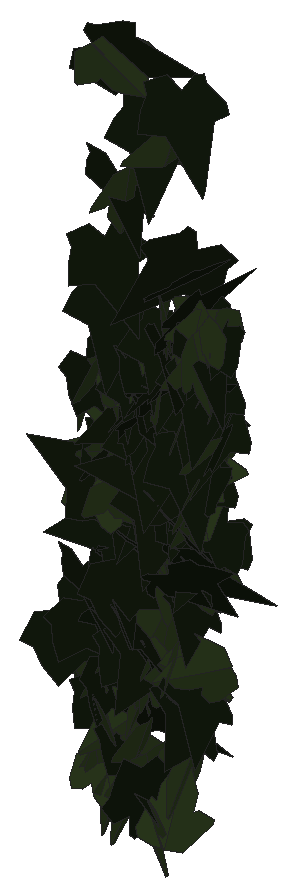
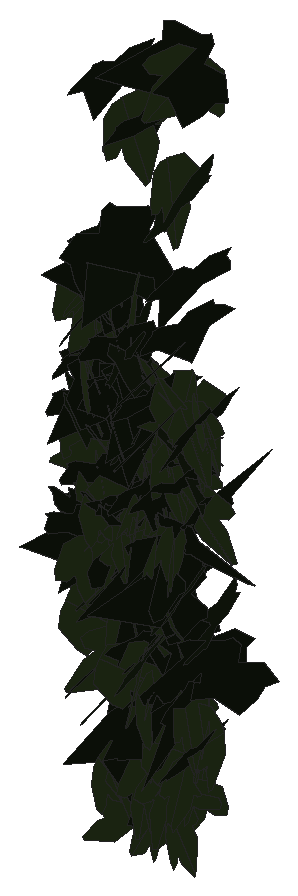
# SketchUp Ruby script. Lengths in inches.
U = 1.inch
M = Sketchup.active_model
def pt(a) = Geom::Point3d.new(a.map { |v| v * U })
def face(e, loops, mat)
  f = e.add_face(loops[0].map { |a| pt(a) })
  loops[1..].each { |l| e.add_face(l.map { |a| pt(a) }).erase! }
  f.material = f.back_material = mat if mat
  f
end
# faces: each face lists its corners as indices into pts; further lists are holes
def faces(e, pts, list, mat = nil) = list.each { |f| face(e, (f[0].is_a?(Array) ? f : [f]).map { |l| l.map { |i| pts[i] } }, mat) }
# xy, xz, yz: faces in a plane at the given z, y or x. An outline is a flat list of corners, or four numbers for a rectangle; further outlines are holes
def ring(l) = l.size == 4 ? [[l[0], l[1]], [l[2], l[1]], [l[2], l[3]], [l[0], l[3]]] : l.each_slice(2).to_a
def flat(e, list, mat, &to3) = list.each { |f| face(e, (f[0].is_a?(Array) ? f : [f]).map { |l| ring(l).map { |u, v| to3.(u, v) } }, mat) }
def xy(e, z, list, mat = nil) = flat(e, list, mat) { |x, y| [x, y, z] }
def xz(e, y, list, mat = nil) = flat(e, list, mat) { |x, z| [x, y, z] }
def yz(e, x, list, mat = nil) = flat(e, list, mat) { |y, z| [x, y, z] }
def lines(e, pts, list) = list.each { |a, b| e.add_line(pt(pts[a]), pt(pts[b])) }
# prism: a flat outline (further loops are holes) pulled along v
def prism(e, loops, v, mat = nil)
  f = face(e, loops, mat); d = Geom::Vector3d.new(v.map { |x| x * U })
  f.pushpull(f.normal.samedirection?(d) ? d.length : -d.length)
end
def box(e, o, s, mat = nil) = prism(e, [[o, [o[0] + s[0], o[1], o[2]], [o[0] + s[0], o[1] + s[1], o[2]], [o[0], o[1] + s[1], o[2]]]], [0, 0, s[2]], mat)
def at(x, y, z, deg = 0) = Geom::Transformation.translation(pt([x, y, z])) * Geom::Transformation.rotation(ORIGIN, Z_AXIS, deg.degrees)
def axes(o, x, y, z) = Geom::Transformation.new([*x, 0, *y, 0, *z, 0, *pt(o).to_a, 1])
def part(name) = M.definitions.add(name)
# library, detail: a bought-in or finely detailed component or shape, given as its bounding box
def library(name, o, s) = part(name).tap { |d| box(d.entities, o, s) }
def detail(e, o, s) = box(e.add_group.entities, o, s)
def put(e, d, t, mat = nil) = e.add_instance(d, t).tap { |i| i.material = mat if mat }
def group(e, t, mat = nil) = e.add_group.tap { |g| g.transformation = t; g.material = mat if mat }.entities
root = M.entities
M.materials.add("efeu1").color = [18, 25, 13]
M.materials.add("efeu2").color = [43, 57, 29]
c1 = part("ivyleaf_9")
p = [[1.54,2.16,1.25],[1.36,2.04,1.19],[-0.21,0.99,0.68],[-0.71,1.11,0.82],[-0.85,0.86,0.67],[-0.8,0.17,0.21],
  [-0.9,-0.01,0.1],[-0.67,-0.16,-0.02],[-0.08,-0.08,-0.05],[-0.03,-0.6,-0.4],[0.65,-0.88,-0.66],[0.83,-0.6,-0.49],
  [1.29,-0.42,-0.43],[1.8125,-0.07,-0.26],[1.21,0.44,0.15]]
faces(c1.entities,p,[[0,1,2,3,4,5,6,7,8,9,10,11,12,13,14]],"efeu1")
c2 = part("ivyleaf_10")
p = [[0,0.5,-0.03],[-0.0625,2.02,-0.43],[-0.19,2.01,-0.46],[-0.54,1.05,-0.29],[-0.52,0.625,-0.18],[-0.83,0.76,-0.28],
  [-1.16,0.64,-0.33],[-1.15,0.33,-0.24],[-0.77,-0.39,0.02],[-0.3,-0.51,0.16],[0.04,-0.48,0.23],[-0.02,2.01,-0.4375],
  [-0.06,2.01,-0.43],[0.04,-0.49,0.23],[0.67,-0.49,0.14],[1.38,0.36,-0.2],[1.375,0.51,-0.24],[0.81,0.65,-0.19],
  [0.62,0.59,-0.15],[0.6,1.09,-0.28],[0.5,1.23,-0.31]]
faces(c2.entities,p,[[0,1,2,3,4,5,6,7,8,9,10],[11,12,0,13,14,15,16,17,18,19,20]],"efeu2")
put(root,c1,axes([527.8,135.33,192.03],[-0.03574,-0.7717,-0.11443],[0.021,-0.11546,0.77209],[-0.77985,0.03225,0.02603]))
put(root,c2,axes([528.8125,134.72,192.54],[-0.44969,-0.49073,-0.36968],[0.25288,0.26967,-0.6656],[0.55993,-0.5159,0.00372]))
put(root,c1,axes([529.75,135.24,194.07],[-0.50214,-0.56983,-0.24591],[0.18261,0.16666,-0.75908],[0.59315,-0.53371,0.02551]))
put(root,c1,axes([529.15,135.53,188.14],[-0.1899,-0.62733,0.39079],[-0.02208,-0.39849,-0.65041],[0.73876,-0.17316,0.08101]))
put(root,c1,axes([530.28,135.32,192.99],[-0.40472,-0.05704,0.74689],[-0.72954,-0.16255,-0.40773],[0.16991,-0.8338,0.02839]))
put(root,c1,axes([530.52,135.21,193.8125],[0.00337,-0.78001,-0.14313],[0.01316,0.14317,-0.7799],[0.79293,0.00094,0.01355]))
put(root,c2,axes([529.96,135.16,201.61],[-0.17501,-0.81085,0.17773],[-0.03106,-0.17511,-0.8295],[0.82952,-0.17762,0.00644]))
put(root,c1,axes([530.56,134.53,190.9],[0.64926,0.46368,0.09757],[0.0766,0.06063,-0.79782],[-0.4676,0.65375,0.00479]))
put(root,c1,axes([529.5,135.23,191.96],[0.37439,-0.43591,0.54064],[0.42975,-0.33705,-0.56937],[0.54555,0.56467,0.0775]))
put(root,c2,axes([531.26,135.26,188.42],[-0.21255,-0.15598,0.72531],[-0.58518,-0.42853,-0.26365],[0.45604,-0.62259,-0.00025]))
put(root,c1,axes([529.3125,135.04,194.65],[-0.69836,0.30086,0.13229],[-0.12525,0.04361,-0.76035],[-0.30386,-0.70944,0.00936]))
put(root,c1,axes([529.4,135.41,201.91],[-0.07236,-0.80977,0.03417],[0.00042,-0.03434,-0.81298],[0.81049,-0.07228,0.00347]))
put(root,c2,axes([528.15,134.8125,186.65],[-0.56665,0.37683,0.32052],[-0.27282,0.16852,-0.68044],[-0.41268,-0.62883,0.00972]))
put(root,c2,axes([528.79,135.09,200.41],[-0.01641,-0.81,-0.0689],[0.01851,0.06853,-0.80999],[0.81271,-0.01792,0.01705]))
put(root,c2,axes([529.46,135.15,195.1875],[0.62857,-0.48335,-0.03124],[-0.01441,0.0325,-0.79274],[0.48415,0.62851,0.01697]))
put(root,c1,axes([528.2,135.48,189.92],[0.22228,-0.68125,0.31969],[0.12627,-0.29486,-0.71612],[0.74186,0.25431,0.0261]))
put(root,c2,axes([528.87,135.4,184.65],[0.09663,-0.71428,0.33007],[0.05891,-0.32505,-0.72066],[0.78465,0.11237,0.01346]))
put(root,c1,axes([528.18,135.52,200.06],[0.20878,-0.72157,0.37063],[0.22611,-0.31578,-0.74215],[0.77905,0.28503,0.11607]))
put(root,c1,axes([527.26,135.44,189.51],[0.33011,-0.63873,0.28091],[0.15388,-0.23647,-0.71852],[0.6806,0.36327,0.02621]))
put(root,c1,axes([529.67,135.69,195.72],[0.08238,-0.52453,0.64775],[0.19724,-0.62015,-0.52726],[0.80982,0.2044,0.06253]))
put(root,c1,axes([528.21,135.5,196.98],[-0.16926,-0.77638,-0.03937],[-0.00605,0.04161,-0.79448],[0.77735,-0.16873,-0.01476]))
put(root,c2,axes([528.55,135.12,192.94],[-0.7037,-0.23781,0.16983],[-0.15629,-0.06789,-0.74267],[0.24691,-0.72071,0.01392]))
put(root,c1,axes([528.42,135.22,185.6],[0.47955,-0.61319,-0.08546],[-0.04016,0.07706,-0.77828],[0.61781,0.48098,0.01574]))
put(root,c2,axes([529.01,135.33,185.88],[0.1496,-0.73188,0.13676],[0.02028,-0.13544,-0.74698],[0.74427,0.1508,-0.00714]))
put(root,c2,axes([530.97,134.96,196.69],[-0.02522,0.77112,0.12282],[-0.07199,0.12006,-0.7686],[-0.77751,-0.03613,0.06718]))
put(root,c2,axes([530.94,135.2,197.25],[-0.6481,0.13698,0.41878],[-0.44061,-0.2064,-0.61436],[0.00291,-0.74351,0.2477]))
put(root,c1,axes([528.87,135.18,189.05],[0.53224,-0.54154,-0.08727],[-0.03394,0.08886,-0.75837],[0.54748,0.53198,0.03783]))
put(root,c1,axes([528.63,134.71,193.51],[-0.18466,0.65837,0.36688],[-0.17846,0.3288,-0.67985],[-0.73226,-0.24616,0.07316]))
put(root,c1,axes([530.18,135.77,186.69],[-0.14093,-0.58061,0.4936],[0.04433,-0.50736,-0.58415],[0.76078,-0.07799,0.12547]))
put(root,c1,axes([530.22,135.33,202.95],[0.02757,-0.77223,-0.27105],[-0.00509,0.27104,-0.77271],[0.8184,0.0277,0.00433]))
put(root,c2,axes([527.68,135.34,194.95],[0.30123,-0.76115,0.04639],[0.00648,-0.04732,-0.81852],[0.76254,0.30109,-0.01137]))
put(root,c1,axes([529.29,134.66,184.28],[-0.0796,-0.05712,0.82665],[0.53853,0.62759,0.09522],[-0.62976,0.54389,-0.02306]))
put(root,c1,axes([529.5625,135.63,192.18],[-0.27612,-0.72698,0.016],[-0.00639,-0.01468,-0.77765],[0.72713,-0.2762,-0.00076]))
put(root,c1,axes([529.32,135.51,194.09],[0.38919,-0.65365,0.20644],[0.10684,-0.17665,-0.76074],[0.6771,0.40358,0.00138]))
put(root,c1,axes([529.83,135.41,195.76],[-0.6008,0.40455,-0.30162],[0.15522,-0.29809,-0.70898],[-0.48015,-0.60256,0.14822]))
put(root,c1,axes([528.67,135.3,191.36],[-0.65059,0.20394,0.39045],[-0.38126,0.08812,-0.68131],[-0.22064,-0.75363,0.02599]))
put(root,c2,axes([530.72,135.125,192.99],[0.21409,-0.69798,-0.30106],[-0.09706,0.28512,-0.73003],[0.75392,0.23491,-0.00849]))
put(root,c1,axes([528.82,135.125,189.24],[0.29871,0.59046,-0.43472],[-0.1676,-0.402,-0.66118],[-0.71382,0.34147,-0.02668]))
put(root,c2,axes([528.78,135.74,187.31],[-0.23096,-0.13339,0.70643],[0.49844,-0.56441,0.05638],[0.51807,0.48356,0.26069]))
put(root,c1,axes([527.98,135.33,198.36],[0.12095,-0.72043,-0.33191],[-0.00905,0.33448,-0.72929],[0.79316,0.11367,0.04229]))
put(root,c2,axes([529.62,135.37,187.98],[-0.62672,-0.06817,0.37557],[-0.33347,-0.25357,-0.60248],[0.18575,-0.68522,0.18558]))
put(root,c2,axes([528.01,135.2,184.92],[0.62327,0.30802,0.18403],[0.13473,0.14096,-0.69223],[-0.33255,0.6344,0.06446]))
put(root,c1,axes([530.4,135.75,187.49],[0.01709,-0.72583,0.23978],[0.06211,-0.23773,-0.72405],[0.76188,0.03566,0.05365]))
put(root,c2,axes([528.49,135.77,186.08],[-0.19638,-0.27838,0.66925],[-0.1969,-0.64681,-0.32682],[0.69758,-0.26094,0.09615]))
put(root,c1,axes([530.08,135.8,189.84],[0.01547,-0.69659,0.34377],[0.11071,-0.33835,-0.69059],[0.76887,0.06274,0.09253]))
put(root,c2,axes([528.16,135.1,203.41],[-0.61065,-0.2846,-0.48513],[0.4563,0.16799,-0.67291],[0.32884,-0.76159,0.03286]))
put(root,c2,axes([530.76,135.375,196.18],[-0.16071,-0.7675,0.0093],[0.05542,-0.02108,-0.78196],[0.76555,-0.15959,0.05856]))
put(root,c2,axes([529.125,135.32,183.92],[-0.54492,0.40266,-0.30524],[0.24575,-0.18104,-0.67755],[-0.44149,-0.59777,-0.00041]))
put(root,c1,axes([530.65,135.76,195.65],[-0.13892,-0.7766,0.1023],[0.00037,-0.10396,-0.78871],[0.78331,-0.13768,0.01851]))
put(root,c1,axes([530.24,135.72,198.67],[-0.07385,0.24379,-0.83335],[-0.04121,-0.8364,-0.24103],[-0.8673,0.01899,0.08241]))
put(root,c2,axes([527.29,135.47,186.63],[-0.46161,0.35338,-0.58612],[0.46446,-0.35751,-0.58135],[-0.50268,-0.65484,0.00108]))
put(root,c2,axes([529.75,135.23,197.25],[-0.49673,0.63448,0.0429],[-0.13759,-0.05409,-0.79328],[-0.62087,-0.49564,0.14148]))
put(root,c1,axes([528.8,134.82,190.55],[0.29483,-0.24248,-0.87086],[-0.01335,0.91474,-0.25922],[0.90389,0.0926,0.28023]))
put(root,c1,axes([528.95,135.73,194.99],[-0.17651,-0.75548,0.0174],[-0.00445,-0.01683,-0.77582],[0.75566,-0.17656,-0.00051]))
put(root,c2,axes([529.47,135.49,188.99],[-0.50086,-0.48174,0.2918],[-0.19998,-0.21293,-0.6948],[0.52652,-0.53913,0.01368]))
put(root,c2,axes([530.94,135.54,197.15],[-0.34051,-0.70121,0.17409],[0.05839,-0.21853,-0.76602],[0.72014,-0.31385,0.14443]))
put(root,c2,axes([530.03,135.16,188.7],[0.40823,-0.5559,-0.49614],[-0.30105,0.39444,-0.68965],[0.68158,0.50718,-0.00745]))
put(root,c1,axes([530.57,135.65,196.76],[0.2515,-0.75774,0.05383],[0.00247,-0.05589,-0.79824],[0.75965,0.25105,-0.01522]))
put(root,c2,axes([528.37,135.21,194.74],[0.68537,-0.10734,0.38785],[-0.37697,0.09688,0.69296],[-0.14086,-0.78152,0.03263]))
put(root,c1,axes([528.62,135.14,188.43],[0.6498,0.10918,-0.4395],[-0.43013,-0.09161,-0.65872],[-0.14163,0.7791,-0.01587]))
put(root,c2,axes([528.6,134.97,192.38],[0.35563,0.39365,0.6463],[0.35924,0.54069,-0.52701],[-0.66604,0.50182,0.06084]))
put(root,c2,axes([528.74,135.5,191.49],[-0.55508,0.30851,-0.44186],[0.32425,-0.31547,-0.62759],[-0.43044,-0.63548,0.09704]))
put(root,c1,axes([527.59,135.11,188.875],[-0.00469,-0.3709,-0.69976],[0.03675,0.69891,-0.3707],[0.79112,-0.03466,0.01307]))
put(root,c2,axes([528.04,135.29,194.47],[0.65068,-0.35549,-0.26657],[-0.14985,0.26945,-0.72509],[0.4183,0.6495,0.15491]))
put(root,c1,axes([529.46,134.81,194.62],[0.27935,0.64425,0.33928],[0.12309,0.31637,-0.70211],[-0.71764,0.30504,0.01164]))
put(root,c2,axes([529.08,135.3125,193.42],[0.53184,-0.50481,-0.2839],[-0.13896,0.26295,-0.72789],[0.56224,0.54251,0.08864]))
put(root,c1,axes([528.01,135.02,203.5625],[0.16967,0.23859,-0.77992],[0.44244,0.64229,0.29274],[0.68516,-0.47384,0.0041]))
put(root,c2,axes([527.83,135.46,192.5],[0.67893,-0.09891,-0.43903],[-0.4333,0.07104,-0.68606],[0.1216,0.80538,0.0066]))
put(root,c2,axes([529.36,135.3,190.87],[-0.62429,0.42429,0.02489],[-0.0211,0.01322,-0.75482],[-0.4245,-0.62464,0.00093]))
put(root,c2,axes([530.85,135.63,195.4],[0.5442,-0.57311,0.1023],[0.05742,-0.08651,-0.79012],[0.57933,0.54693,-0.01779]))
put(root,c2,axes([530.04,135.06,190.37],[-0.12901,0.63164,0.40942],[-0.13435,0.38939,-0.64309],[-0.74064,-0.18066,0.04534]))
put(root,c1,axes([526.98,135.09,188.48],[0.26067,-0.27434,-0.85378],[0.2872,0.86783,-0.19116],[0.84954,-0.20921,0.3266]))
put(root,c1,axes([530.87,135.06,192.67],[-0.72338,0.34776,-0.12421],[-0.11613,0.04509,0.80258],[0.35054,0.73258,0.00956]))
put(root,c1,axes([530.35,134.85,197.2],[-0.09302,0.65707,-0.46318],[-0.09984,0.45322,0.66299],[0.79769,0.13335,0.02897]))
put(root,c1,axes([530.2,135.32,190.64],[0.62236,-0.07483,0.49451],[0.49263,-0.04458,-0.62674],[0.08635,0.79365,0.01142]))
put(root,c2,axes([528.78,135.97,187.24],[0.1445,-0.54934,0.56919],[0.26502,-0.51155,-0.56099],[0.74533,0.2884,0.08912]))
put(root,c1,axes([531.12,135.71,197],[-0.75984,0.03985,-0.22383],[0.22384,-0.00565,-0.76086],[-0.03982,-0.7921,-0.00583]))
put(root,c2,axes([528.18,135.35,194],[0.75951,0.16265,-0.27372],[0.26857,0.05298,0.77672],[0.17101,-0.80558,-0.00418]))
put(root,c2,axes([529.85,135.74,194.0625],[0.43704,-0.62924,0.18954],[0.1091,-0.155,-0.76612],[0.64805,0.45045,0.00115]))
put(root,c1,axes([529.67,135.875,196.27],[-0.37369,-0.68913,-0.10923],[0.06432,0.08936,-0.78381],[0.69476,-0.37893,0.01381]))
put(root,c2,axes([529.24,135.46,193.21],[0.37908,-0.62975,-0.27747],[-0.15115,0.23285,-0.73499],[0.67136,0.408,-0.00881]))
put(root,c1,axes([530.65,135.93,194.58],[-0.40838,-0.67211,-0.04345],[0.01731,0.04032,-0.78643],[0.67329,-0.4087,-0.00614]))
put(root,c2,axes([527.92,135.59,187.25],[0.09212,-0.74944,-0.06245],[-0.00056,0.06285,-0.75505],[0.75204,0.09185,0.00709]))
put(root,c1,axes([528.57,135.43,190.47],[0.73295,-0.16802,0.24714],[0.24013,-0.05855,-0.75196],[0.1779,0.77128,-0.00324]))
put(root,c2,axes([528.31,135.6875,193.55],[-0.05562,-0.77626,0.0687],[0.02045,-0.0703,-0.77784],[0.77903,-0.05358,0.02532]))
put(root,c2,axes([530.68,135.47,192.38],[0.04575,-0.7902,-0.24837],[0.01383,0.24944,-0.79106],[0.8282,0.03949,0.02693]))
put(root,c1,axes([528.8125,135.46,188.43],[-0.04116,-0.51639,-0.61805],[0.14448,0.60408,-0.51434],[0.79232,-0.13698,0.06168]))
put(root,c1,axes([527.38,135.47,194.96],[0.40294,-0.55665,-0.39636],[-0.12426,0.39278,-0.67795],[0.67196,0.40643,0.11231]))
put(root,c2,axes([530.58,135.4375,196.77],[-0.48192,0.36232,0.49663],[-0.5447,0.04088,-0.55839],[-0.285,-0.69081,0.22743]))
put(root,c1,axes([528.85,135.68,195.59],[0.36429,-0.67624,-0.17594],[0.0172,0.20703,-0.76013],[0.69854,0.34757,0.11047]))
put(root,c2,axes([528.3,135.73,189.13],[0.50551,-0.07101,0.60035],[0.60087,-0.02705,-0.50914],[0.06648,0.78437,0.0368]))
put(root,c2,axes([530.1875,135.99,191.92],[-0.0329,-0.6402,0.41441],[0.02916,-0.41555,-0.63964],[0.76207,-0.01174,0.04237]))
put(root,c2,axes([529.07,135.5,185.125],[-0.2856,-0.66197,-0.21211],[0.0746,0.1988,-0.72089],[0.69111,-0.29502,-0.00984]))
put(root,c2,axes([530.9,135.79,193.78],[-0.02475,-0.77514,0.11777],[-0.01472,-0.11735,-0.77546],[0.7839,-0.02668,-0.01085]))
put(root,c2,axes([527.96,135.89,184.26],[0.14886,-0.65289,0.25509],[0.10371,-0.2374,-0.66812],[0.69324,0.17571,0.04518]))
put(root,c2,axes([529.95,135.32,187.93],[-0.3966,-0.30421,-0.61536],[0.50503,0.35203,-0.49952],[0.46493,-0.6419,0.01769]))
put(root,c1,axes([531.02,135.82,194.27],[-0.59835,0.31608,-0.38321],[0.31906,-0.21527,-0.67575],[-0.38073,-0.67715,0.03595]))
put(root,c1,axes([529.76,135.85,191.64],[0.29597,-0.69904,-0.00213],[0.03799,0.0184,-0.75794],[0.69801,0.29541,0.04216]))
put(root,c2,axes([528.27,135.51,185.18],[-0.52329,-0.55975,-0.22734],[0.1574,0.16407,-0.76625],[0.58329,-0.54644,0.00281]))
put(root,c1,axes([527.53,135.75,186.37],[0.26491,-0.68887,-0.20091],[-0.03503,0.20149,-0.73706],[0.71672,0.26447,0.03823]))
put(root,c2,axes([529.27,135.34,187.83],[0.21716,-0.55667,-0.48039],[0.0646,0.51341,-0.56573],[0.73245,0.11976,0.19232]))
put(root,c1,axes([528.77,136.12,192.9],[-0.15884,-0.75624,0.07728],[0.00173,-0.07931,-0.77254],[0.76018,-0.15784,0.0179]))
put(root,c1,axes([529.5,135.41,194.9],[0.39583,0.6132,-0.26896],[-0.16616,-0.21271,-0.7295],[-0.64865,0.42869,0.02275]))
put(root,c1,axes([530.15,136.05,192.91],[-0.46291,-0.60795,-0.10425],[0.07368,0.07492,-0.76401],[0.61241,-0.46855,0.01311]))
put(root,c2,axes([530.5625,135.82,195.08],[0.28588,-0.73114,0.05065],[0.04811,-0.03552,-0.7844],[0.73131,0.28815,0.03181]))
put(root,c2,axes([527.96,135.52,194.625],[0.64806,-0.02833,-0.40706],[-0.35916,0.323,-0.59427],[0.19367,0.69379,0.26004]))
put(root,c1,axes([527.95,135.37,187.43],[0.33319,-0.39721,-0.66676],[-0.39399,0.5386,-0.51774],[0.66867,0.51527,0.02718]))
put(root,c1,axes([528.81,136.31,193.9],[-0.18848,-0.55904,0.48848],[0.014,-0.50656,-0.57433],[0.74225,-0.1324,0.13487]))
put(root,c2,axes([527.94,135.95,191.41],[0.17968,-0.6482,0.33945],[0.40655,-0.20217,-0.60127],[0.60836,0.32655,0.30154]))
put(root,c2,axes([529.25,135.73,192.31],[-0.24266,0.69755,-0.19782],[0.02686,-0.19981,-0.73753],[-0.72456,-0.24103,0.03891]))
put(root,c2,axes([530.6,135.73,190.38],[-0.55669,-0.4853,0.09085],[-0.06432,-0.06447,-0.7385],[0.48952,-0.56036,0.00629]))
put(root,c1,axes([528.13,135.34,189.98],[0.61766,0.0895,0.47053],[0.45259,0.14223,-0.62117],[-0.15675,0.76333,0.06057]))
put(root,c1,axes([530.91,135.96,191.71],[-0.75409,-0.12576,-0.12036],[0.11592,0.03639,-0.76433],[0.12986,-0.76277,-0.01662]))
put(root,c1,axes([528.9,135.41,186.55],[0.78172,0.09078,0.29446],[0.29302,0.02943,-0.78696],[-0.09534,0.83482,-0.00428]))
put(root,c2,axes([528,135.57,185.48],[-0.08029,-0.65111,-0.29642],[0.12709,0.28056,-0.65069],[0.70403,-0.1249,0.08365]))
put(root,c1,axes([530.0625,135.14,198],[0.35776,0.63808,0.28206],[-0.03798,0.33433,-0.70815],[-0.6966,0.30948,0.18346]))
put(root,c2,axes([529.72,135.39,183.66],[0.38243,0.66246,-0.36227],[0.15296,0.3297,0.76436],[0.73939,-0.41085,0.02925]))
put(root,c2,axes([529.97,135.65,191.54],[-0.64402,0.18696,0.35491],[-0.36196,0.0185,-0.66657],[-0.1729,-0.7351,0.07349]))
put(root,c1,axes([528,135.97,193.12],[0.0122,-0.74967,-0.23177],[0.04368,0.23208,-0.7484],[0.78347,-0.00127,0.04533]))
put(root,c1,axes([530.18,135.27,194.91],[0.50479,0.51406,0.27066],[0.2074,0.17547,-0.72008],[-0.54267,0.54524,-0.02344]))
put(root,c1,axes([530.63,136.2,191.53],[-0.55338,-0.53924,-0.0067],[0.02318,-0.01419,-0.77222],[0.53879,-0.55324,0.02634]))
put(root,c2,axes([529.56,136.13,187.91],[-0.2738,-0.07845,0.70308],[-0.48654,-0.52641,-0.24821],[0.51357,-0.54053,0.13969]))
put(root,c1,axes([528.67,136.15,188.51],[0.26159,-0.68256,0.21834],[0.09617,-0.19689,-0.73074],[0.71015,0.27809,0.01853]))
put(root,c2,axes([530.22,135.7,193.0625],[0.51359,0.65355,0.1581],[0.10536,0.11827,-0.83115],[-0.6641,0.5242,-0.0096]))
put(root,c2,axes([529.73,136.23,185.32],[0.01452,-0.60516,0.47972],[0.20286,-0.45996,-0.58638],[0.74511,0.13702,0.1503]))
